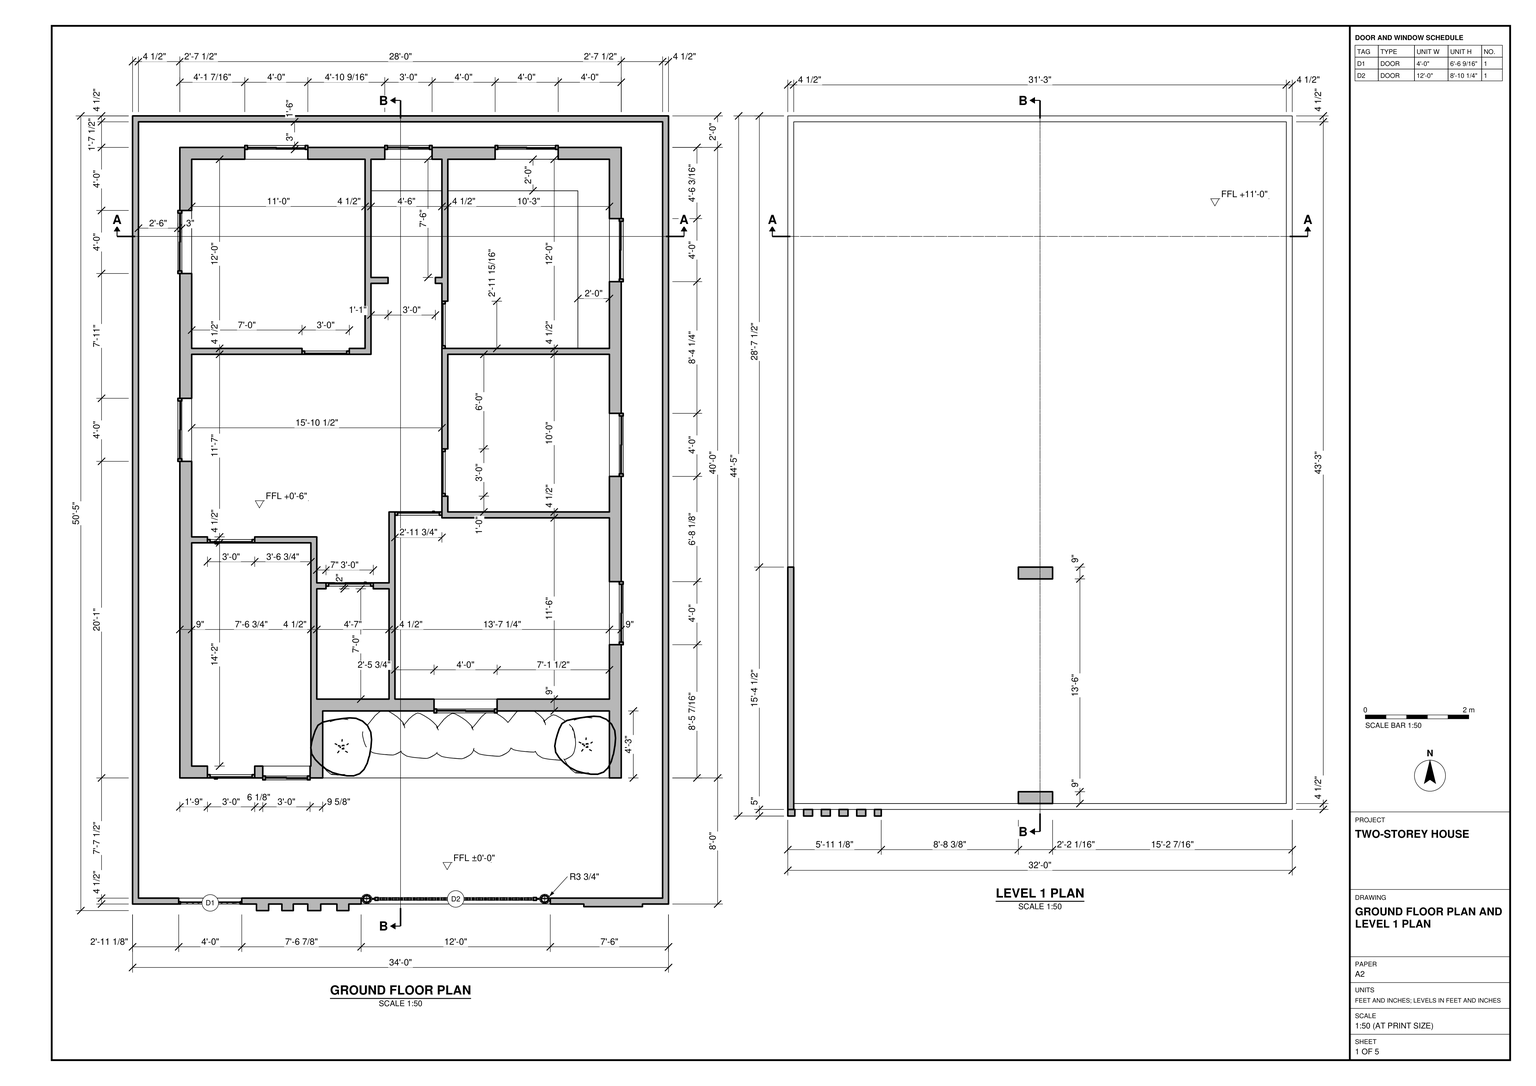
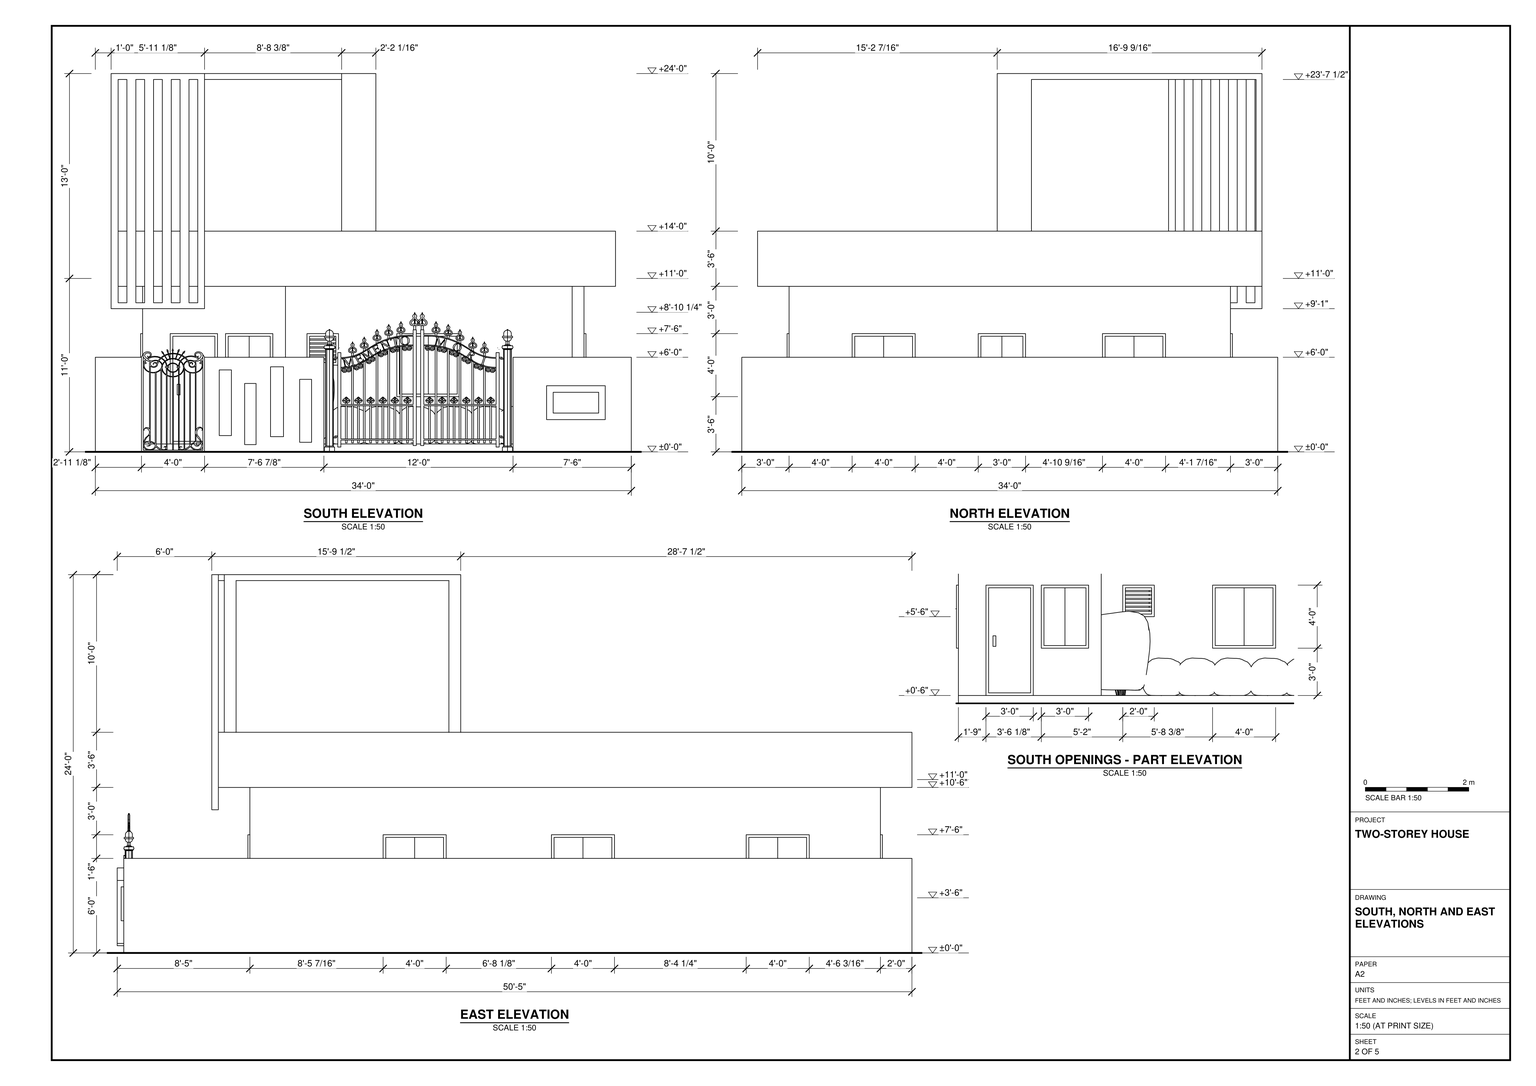
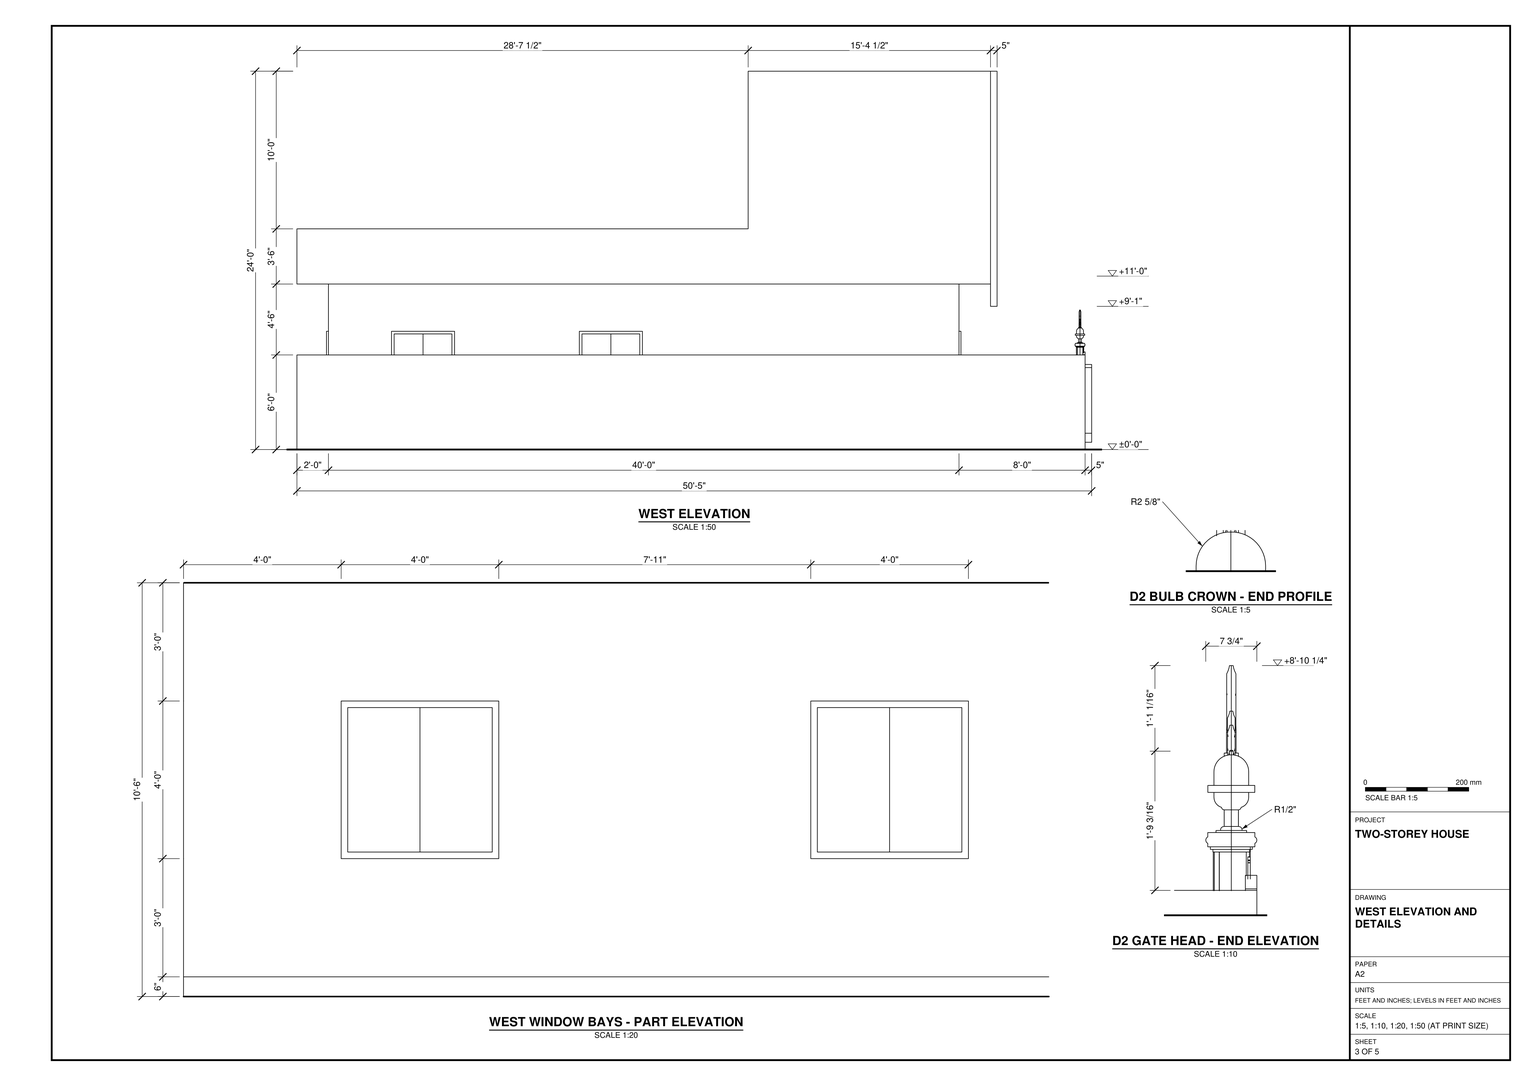
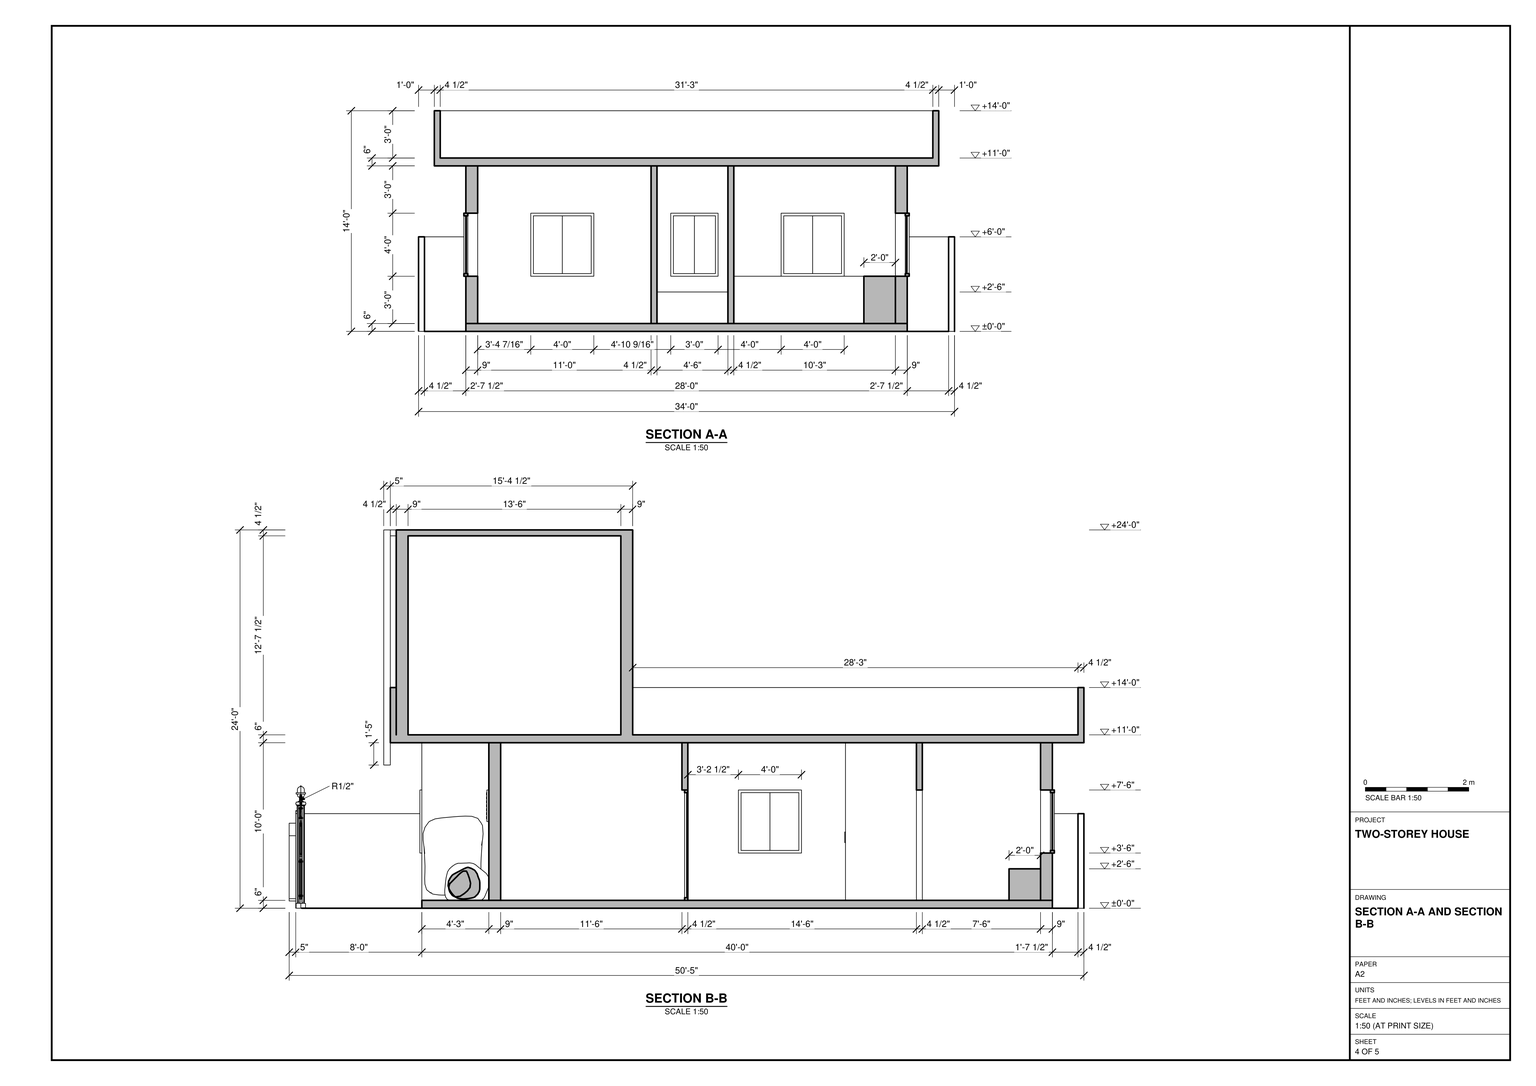
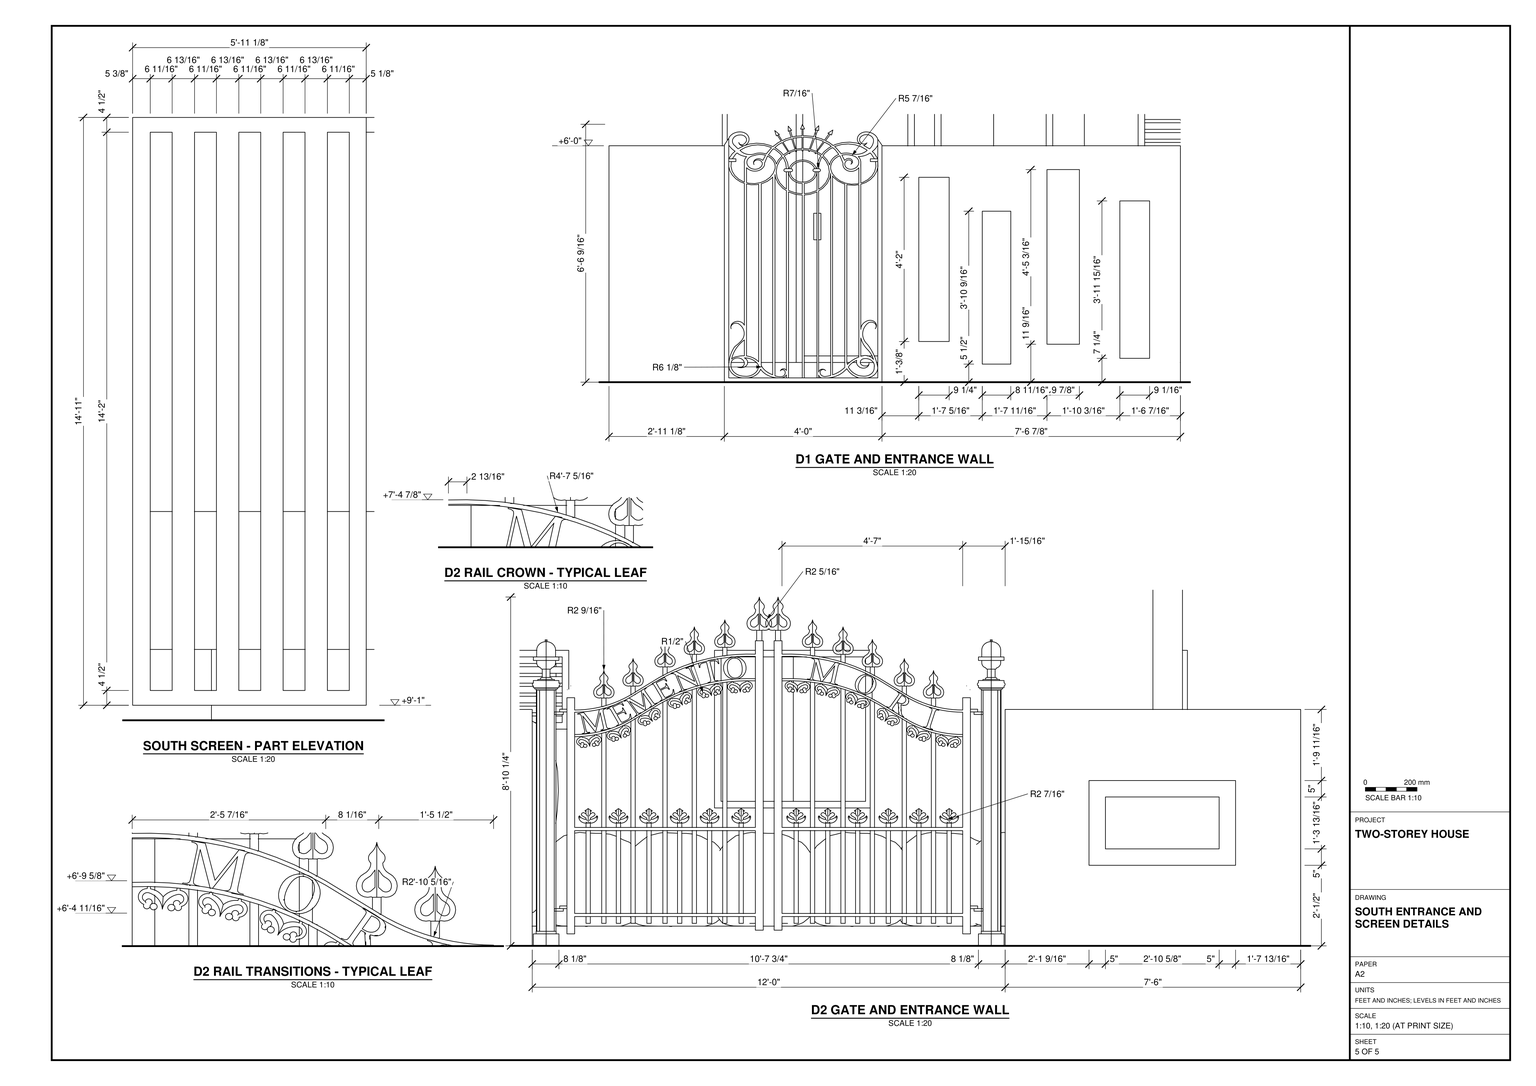
Build the house and its walled site in SketchUp using task_files/diagram_01.pdf. Work in feet and inches. The overall model is 34'-0" wide, 50'-5" deep and 24'-0" high. Use ±0'-0" as the ground datum and +11'-0" as the upper level. Set the house floor at +0'-6", above the forecourt.

Lay out the house behind the south boundary wall, leaving the forecourt, side clearances and rear setback shown in plan. Model the 9" exterior house walls and 4 1/2" interior partitions. Follow the room divisions, connecting doorways and framed window openings on the plan and elevations. At the front, distinguish the projecting entrance room from the recessed wall and planting strip beside it. Build the flat slab over the ground floor, the parapet around the open terrace and the tall frame with vertical fins at the southwest corner.

Model the narrow pedestrian gate and wider double gate in the south boundary wall. Use the elevations to shape the gate heads and place the panels in the adjoining wall. Decor and loose items, including the planting, may use any suitable library components. Keep shell elements such as walls, slabs and roof separate as groups or components, do the same for each furniture or joinery piece, and use components for repeated parts. Save one SketchUp model as output_files/two_storey_house_with_roof_terrace_and_gated_forecourt.skp.

# SketchUp Ruby script. Lengths in inches.
U = 1.inch
M = Sketchup.active_model
def pt(a) = Geom::Point3d.new(a.map { |v| v * U })
def face(e, loops, mat)
  f = e.add_face(loops[0].map { |a| pt(a) })
  loops[1..].each { |l| e.add_face(l.map { |a| pt(a) }).erase! }
  f.material = f.back_material = mat if mat
  f
end
# faces: each face lists its corners as indices into pts; further lists are holes
def faces(e, pts, list, mat = nil) = list.each { |f| face(e, (f[0].is_a?(Array) ? f : [f]).map { |l| l.map { |i| pts[i] } }, mat) }
# xy, xz, yz: faces in a plane at the given z, y or x. An outline is a flat list of corners, or four numbers for a rectangle; further outlines are holes
def ring(l) = l.size == 4 ? [[l[0], l[1]], [l[2], l[1]], [l[2], l[3]], [l[0], l[3]]] : l.each_slice(2).to_a
def flat(e, list, mat, &to3) = list.each { |f| face(e, (f[0].is_a?(Array) ? f : [f]).map { |l| ring(l).map { |u, v| to3.(u, v) } }, mat) }
def xy(e, z, list, mat = nil) = flat(e, list, mat) { |x, y| [x, y, z] }
def xz(e, y, list, mat = nil) = flat(e, list, mat) { |x, z| [x, y, z] }
def yz(e, x, list, mat = nil) = flat(e, list, mat) { |y, z| [x, y, z] }
def lines(e, pts, list) = list.each { |a, b| e.add_line(pt(pts[a]), pt(pts[b])) }
# prism: a flat outline (further loops are holes) pulled along v
def prism(e, loops, v, mat = nil)
  f = face(e, loops, mat); d = Geom::Vector3d.new(v.map { |x| x * U })
  f.pushpull(f.normal.samedirection?(d) ? d.length : -d.length)
end
def box(e, o, s, mat = nil) = prism(e, [[o, [o[0] + s[0], o[1], o[2]], [o[0] + s[0], o[1] + s[1], o[2]], [o[0], o[1] + s[1], o[2]]]], [0, 0, s[2]], mat)
def at(x, y, z, deg = 0) = Geom::Transformation.translation(pt([x, y, z])) * Geom::Transformation.rotation(ORIGIN, Z_AXIS, deg.degrees)
def axes(o, x, y, z) = Geom::Transformation.new([*x, 0, *y, 0, *z, 0, *pt(o).to_a, 1])
def part(name) = M.definitions.add(name)
# library, detail: a bought-in or finely detailed component or shape, given as its bounding box
def library(name, o, s) = part(name).tap { |d| box(d.entities, o, s) }
def detail(e, o, s) = box(e.add_group.entities, o, s)
def put(e, d, t, mat = nil) = e.add_instance(d, t).tap { |i| i.material = mat if mat }
def group(e, t, mat = nil) = e.add_group.tap { |g| g.transformation = t; g.material = mat if mat }.entities
root = M.entities
M.materials.add("Aluminium Black Anodized Fingerprints 15cm").color = [38, 38, 38]
M.materials.add("Glass Coated Blue").color = [0, 0, 0]
M.materials["Glass Coated Blue"].alpha = 0.35
M.materials.add("Grass C 200cm").color = [118, 136, 72]
M.materials.add("Tiles K01 100cm").color = [149, 135, 123]
M.materials.add("Wall Paint Fine Grain 01 Yellow 100cm").color = [207, 190, 139]
M.materials.add("Wall Paint Poised Taupe Satin 300cm").color = [140, 135, 132]
M.materials.add("Wood Dark 02 100cm").color = [99, 39, 19]
M.materials.add("Wood Dark Fine 18-26 80cm").color = [104, 73, 63]
c1 = library("Schefflera arboricola 001",[-25.43,-22.82,-0.1],[47.76,45.73,64.24])
c2 = library("Skimmia japonica Rubella 004",[-17.08,-16.64,-0.26],[33.2,34.59,28.81])
c3 = library("gate 533k",[0,0,0],[7.78,132.3,106.23])
c4 = library("gate 458k",[0,0,0],[53.16,1.75,104.71])
c5 = library("Dome Light",[-12,-12,0],[24,24,12])
c6 = part("Group\#6")
box(c6.entities,[0,0,0],[16,0.31,44])
c7 = part("Group\#8")
box(c7.entities,[0,-0.31,0],[20,0.31,2])
c8 = part("Group\#10")
box(c8.entities,[0,0,0],[22,0.31,44])
c9 = part("Group\#12")
box(c9.entities,[-0.31,0,0],[0.31,22,44])
c10 = part("Group\#14")
box(c10.entities,[-0.31,0,0],[0.31,22,44])
c11 = part("Group\#16")
box(c11.entities,[-0.31,0,0],[0.31,22,44])
c12 = part("Group\#18")
box(c12.entities,[0,-0.31,0],[22,0.31,44])
c13 = part("Group\#20")
box(c13.entities,[0,-0.31,0],[16,0.31,44])
c14 = part("Group\#22")
box(c14.entities,[0,-0.31,0],[22,0.31,44])
c15 = part("Group\#24")
box(c15.entities,[0,0,0],[0.31,22,44])
c16 = part("Group\#26")
box(c16.entities,[0,0,0],[0.31,22,44])
put(root,c1,at(159.61,124.73,0))
put(root,c1,at(345.35,125.97,0))
put(root,c2,at(192.09,135.07,0))
put(root,c2,at(217.83,132.5,0))
put(root,c2,at(244.47,132.23,0))
put(root,c2,at(273.02,134.13,0))
put(root,c2,at(299.28,137.3,0))
put(root,c2,at(321.125,131.1,0))
put(root,c3,axes([318,12.78,-6],[0,-1,0],[-1.08843,0,0],[0,0,1]))
put(root,c4,axes([35.125,5,-6],[0.90286,0,0],[0,1,0],[0,0,0.75]))
put(root,c5,axes([-74.51,70.32,-1.87],[2.55,0,0],[0,1,0],[0,0,2.51]))
g1 = group(root,at(36,101,0))
xy(g1,0,[[0,0,0,480,336,480,336,0,327,0,327,51,108.75,51,108.75,0,57,0,57,9,99.75,9,99.75,179,57,179,57,183.5,104.25,183.5,104.25,148.5,111.25,148.5,111.25,144,104.25,144,104.25,60,159.25,60,159.25,144,147.25,144,147.25,148.5,159.25,148.5,159.25,202.5,163.75,202.5,163.75,60,327,60,327,198,199.5,198,199.5,214.5,204,214.5,204,202.5,327,202.5,327,322.5,204,322.5,204,250.5,199.5,250.5,199.5,327,327,327,327,471,204,471,204,362.9375,199.5,362.9375,199.5,376.5,194.5,376.5,194.5,381,199.5,381,199.5,471,145.5,471,145.5,381,158.5,381,158.5,376.5,145.5,376.5,145.5,322.5,129,322.5,129,327,141,327,141,471,9,471,9,327,93,327,93,322.5,9,322.5,9,183.5,21,183.5,21,179,9,179,9,9,21,9,21,0]])
xy(g1,36,[[63.125,0,99.125,9],[193.5,51,241.5,60],[327,101.4375,336,149.4375],[327,229.5625,336,277.5625],[0,241,9,289],
  [327,377.8125,336,425.8125],[0,384,9,432],[49.4375,471,97.4375,480],[156,471,192,480],[240,471,288,480]])
xy(g1,60,[[125.125,51,149.125,60]])
xy(g1,84,[[21,0,57,9],[63.125,0,99.125,9],[125.125,51,149.125,60],[193.5,51,241.5,60],[327,101.4375,336,149.4375],
  [111.25,144,147.25,148.5],[21,179,57,183.5],[163.75,198,199.5,202.5],[199.5,214.5,204,250.5],[327,229.5625,336,277.5625],
  [0,241,9,289],[93,322.5,129,327],[199.5,327,204,362.9375],[158.5,376.5,194.5,381],[327,377.8125,336,425.8125],
  [0,384,9,432],[49.4375,471,97.4375,480],[156,471,192,480],[240,471,288,480]])
xy(g1,120,[[[0,0,108.75,0,108.75,51,327,51,327,0,336,0,336,480,0,480],[104.25,148.5,104.25,183.5,9,183.5,9,322.5,145.5,322.5,145.5,376.5,199.5,376.5,199.5,202.5,159.25,202.5,159.25,148.5],[163.75,60,327,198],[9,327,141,471],[204,327,327,471],[9,9,99.75,179],[204,202.5,327,322.5],[145.5,381,199.5,471],[104.25,60,159.25,144]]])
xz(g1,0,[[[0,0,21,0,21,84,57,84,57,0,108.75,0,108.75,120,0,120],[63.125,36,99.125,84]],[327,0,336,120]],"Wall Paint Fine Grain 01 Yellow 100cm")
xz(g1,9,[[[9,0,9,120,99.75,120,99.75,0,57,0,57,84,21,84,21,0],[63.125,36,99.125,84]]])
xz(g1,51,[[[108.75,0,327,120],[193.5,36,241.5,84],[125.125,60,149.125,84]]],"Wall Paint Fine Grain 01 Yellow 100cm")
xz(g1,60,[[[104.25,0,159.25,120],[125.125,60,149.125,84]],[[163.75,0,327,120],[193.5,36,241.5,84]]])
xz(g1,101.4375,[[327,36,336,84]])
xz(g1,144,[[104.25,0,111.25,0,111.25,84,147.25,84,147.25,0,159.25,0,159.25,120,104.25,120]])
xz(g1,148.5,[[104.25,0,104.25,120,159.25,120,159.25,0,147.25,0,147.25,84,111.25,84,111.25,0]])
xz(g1,149.4375,[[327,36,336,84]])
xz(g1,179,[[9,0,21,0,21,84,57,84,57,0,99.75,0,99.75,120,9,120]])
xz(g1,183.5,[[9,0,9,120,104.25,120,104.25,0,57,0,57,84,21,84,21,0]])
xz(g1,198,[[199.5,0,327,0,327,120,163.75,120,163.75,84,199.5,84]])
xz(g1,202.5,[[159.25,0,159.25,120,199.5,120,199.5,84,163.75,84,163.75,0],[204,0,327,120]])
xz(g1,214.5,[[199.5,0,204,84]])
xz(g1,229.5625,[[327,36,336,84]])
xz(g1,241,[[0,36,9,84]])
xz(g1,250.5,[[199.5,0,204,84]])
xz(g1,277.5625,[[327,36,336,84]])
xz(g1,289,[[0,36,9,84]])
xz(g1,322.5,[[9,0,93,0,93,84,129,84,129,0,145.5,0,145.5,120,9,120],[204,0,327,120]])
xz(g1,327,[[9,0,9,120,141,120,141,0,129,0,129,84,93,84,93,0],[199.5,0,199.5,84,204,84,204,120,327,120,327,0]])
xz(g1,362.9375,[[199.5,0,204,84]])
xz(g1,376.5,[[145.5,0,158.5,0,158.5,84,194.5,84,194.5,0,199.5,0,199.5,120,145.5,120]])
xz(g1,377.8125,[[327,36,336,84]])
xz(g1,381,[[145.5,0,145.5,120,199.5,120,199.5,0,194.5,0,194.5,84,158.5,84,158.5,0]])
xz(g1,384,[[0,36,9,84]])
xz(g1,425.8125,[[327,36,336,84]])
xz(g1,432,[[0,36,9,84]])
xz(g1,471,[[[9,0,141,120],[49.4375,36,97.4375,84]],[[145.5,0,199.5,120],[156,36,192,84]],[[204,0,327,120],[240,36,288,84]]])
xz(g1,480,[[[0,0,336,120],[240,36,288,84],[49.4375,36,97.4375,84],[156,36,192,84]]],"Wall Paint Fine Grain 01 Yellow 100cm")
yz(g1,0,[[[0,0,480,120],[384,36,432,84],[241,36,289,84]]],"Wall Paint Fine Grain 01 Yellow 100cm")
yz(g1,9,[[9,0,179,120],[[183.5,0,322.5,120],[241,36,289,84]],[[327,0,471,120],[384,36,432,84]]])
yz(g1,21,[[0,0,9,84],[179,0,183.5,84]])
yz(g1,49.4375,[[471,36,480,84]])
yz(g1,57,[[0,0,9,84],[179,0,183.5,84]])
yz(g1,63.125,[[0,36,9,84]])
yz(g1,93,[[322.5,0,327,84]])
yz(g1,97.4375,[[471,36,480,84]])
yz(g1,99.125,[[0,36,9,84]])
yz(g1,99.75,[[9,0,179,120]])
yz(g1,104.25,[[60,0,144,120],[148.5,0,183.5,120]])
yz(g1,108.75,[[0,0,51,120]],"Wall Paint Fine Grain 01 Yellow 100cm")
yz(g1,111.25,[[144,0,148.5,84]])
yz(g1,125.125,[[51,60,60,84]])
yz(g1,129,[[322.5,0,327,84]])
yz(g1,141,[[327,0,471,120]])
yz(g1,145.5,[[322.5,0,376.5,120],[381,0,471,120]])
yz(g1,147.25,[[144,0,148.5,84]])
yz(g1,149.125,[[51,60,60,84]])
yz(g1,156,[[471,36,480,84]])
yz(g1,158.5,[[376.5,0,381,84]])
yz(g1,159.25,[[60,0,144,120],[148.5,0,202.5,120]])
yz(g1,163.75,[[60,0,202.5,0,202.5,84,198,84,198,120,60,120]])
yz(g1,192,[[471,36,480,84]])
yz(g1,193.5,[[51,36,60,84]])
yz(g1,194.5,[[376.5,0,381,84]])
yz(g1,199.5,[[198,0,198,84,202.5,84,202.5,120,376.5,120,376.5,0,362.9375,0,362.9375,84,327,84,327,0,250.5,0,250.5,84,214.5,84,214.5,0],[381,0,471,120]])
yz(g1,204,[[202.5,0,214.5,0,214.5,84,250.5,84,250.5,0,322.5,0,322.5,120,202.5,120],[362.9375,0,471,0,471,120,327,120,327,84,362.9375,84]])
yz(g1,240,[[471,36,480,84]])
yz(g1,241.5,[[51,36,60,84]])
yz(g1,288,[[471,36,480,84]])
yz(g1,327,[[[60,0,198,120],[101.4375,36,149.4375,84]],[[202.5,0,322.5,120],[229.5625,36,277.5625,84]],[[327,0,471,120],[377.8125,36,425.8125,84]]])
yz(g1,327,[[0,0,51,120]],"Wall Paint Fine Grain 01 Yellow 100cm")
yz(g1,336,[[[0,0,480,120],[377.8125,36,425.8125,84],[101.4375,36,149.4375,84],[229.5625,36,277.5625,84]]],"Wall Paint Fine Grain 01 Yellow 100cm")
g2 = group(g1,at(21,0,0),"Aluminium Black Anodized Fingerprints 15cm")
prism(g2,[[[36,0,0],[36,0,84],[0,0,84],[0,0,0]],[[34,0,82],[34,0,2],[2,0,2],[2,0,82]]],[0,2.5,0],"Aluminium Black Anodized Fingerprints 15cm")
g3 = group(g1,at(23,0,2))
box(g3,[0,0,0],[32,0.71,80],"Wood Dark 02 100cm")
g4 = group(g3,at(3.34,0,35.37),"Aluminium Black Anodized Fingerprints 15cm")
box(g4,[0,-0.75,0],[2.1875,0.75,8.0625],"Aluminium Black Anodized Fingerprints 15cm")
g5 = group(g1,at(63.125,0,36))
prism(g5,[[[36,-1.5,0],[36,-1.5,48],[0,-1.5,48],[0,-1.5,0]],[[2,-1.5,46],[34,-1.5,46],[34,-1.5,2],[2,-1.5,2]]],[0,3,0],"Aluminium Black Anodized Fingerprints 15cm")
put(g5,c6,at(2,0,2),"Glass Coated Blue")
put(g5,c6,at(18,-0.31,2),"Glass Coated Blue")
g6 = group(g1,at(125.125,51,60))
prism(g6,[[[0,-1.5,0],[24,-1.5,0],[24,-1.5,24],[0,-1.5,24]],[[2,-1.5,2],[2,-1.5,22],[22,-1.5,22],[22,-1.5,2]]],[0,3,0],"Aluminium Black Anodized Fingerprints 15cm")
put(g6,c7,at(2,-1.5,20),"Glass Coated Blue")
put(g6,c7,at(2,-1.5,17),"Glass Coated Blue")
put(g6,c7,at(2,-1.5,14),"Glass Coated Blue")
put(g6,c7,at(2,-1.5,11),"Glass Coated Blue")
put(g6,c7,at(2,-1.5,8),"Glass Coated Blue")
put(g6,c7,at(2,-1.5,5),"Glass Coated Blue")
put(g6,c7,at(2,-1.5,2),"Glass Coated Blue")
g7 = group(g1,at(193.5,51,36))
prism(g7,[[[0,-1.5,0],[48,-1.5,0],[48,-1.5,48],[0,-1.5,48]],[[46,-1.5,2],[2,-1.5,2],[2,-1.5,46],[46,-1.5,46]]],[0,3,0],"Aluminium Black Anodized Fingerprints 15cm")
put(g7,c8,at(2,0.0625,2),"Glass Coated Blue")
put(g7,c8,at(24,-0.25,2),"Glass Coated Blue")
g8 = group(g1,at(336,101.4375,36))
prism(g8,[[[1.5,0,0],[1.5,48,0],[1.5,48,48],[1.5,0,48]],[[1.5,46,46],[1.5,46,2],[1.5,2,2],[1.5,2,46]]],[-3,0,0],"Aluminium Black Anodized Fingerprints 15cm")
put(g8,c9,at(0.125,2,2),"Glass Coated Blue")
put(g8,c9,at(0.44,24,2),"Glass Coated Blue")
g9 = group(g1,at(336,229.5625,36))
prism(g9,[[[1.5,0,0],[1.5,48,0],[1.5,48,48],[1.5,0,48]],[[1.5,46,2],[1.5,2,2],[1.5,2,46],[1.5,46,46]]],[-3,0,0],"Aluminium Black Anodized Fingerprints 15cm")
put(g9,c10,at(0,2,2),"Glass Coated Blue")
put(g9,c10,at(0.31,24,2),"Glass Coated Blue")
g10 = group(g1,at(336,377.8125,36))
prism(g10,[[[1.5,48,0],[1.5,48,48],[1.5,0,48],[1.5,0,0]],[[1.5,46,2],[1.5,2,2],[1.5,2,46],[1.5,46,46]]],[-3,0,0],"Aluminium Black Anodized Fingerprints 15cm")
put(g10,c11,at(-0.5625,2,2),"Glass Coated Blue")
put(g10,c11,at(-0.25,24,2),"Glass Coated Blue")
g11 = group(g1,at(240,480,36))
prism(g11,[[[48,1.5,0],[0,1.5,0],[0,1.5,48],[48,1.5,48]],[[46,1.5,46],[2,1.5,46],[2,1.5,2],[46,1.5,2]]],[0,-3,0],"Aluminium Black Anodized Fingerprints 15cm")
put(g11,c12,at(24,-0.3125,2),"Glass Coated Blue")
put(g11,c12,at(2,0,2),"Glass Coated Blue")
g12 = group(g1,at(156,480,36))
prism(g12,[[[0,1.5,0],[0,1.5,48],[36,1.5,48],[36,1.5,0]],[[34,1.5,46],[2,1.5,46],[2,1.5,2],[34,1.5,2]]],[0,-3,0],"Aluminium Black Anodized Fingerprints 15cm")
put(g12,c13,at(18,-0.1875,2),"Glass Coated Blue")
put(g12,c13,at(2,0.13,2),"Glass Coated Blue")
g13 = group(g1,at(49.4375,480,36))
prism(g13,[[[48,1.5,0],[0,1.5,0],[0,1.5,48],[48,1.5,48]],[[2,1.5,2],[46,1.5,2],[46,1.5,46],[2,1.5,46]]],[0,-3,0],"Aluminium Black Anodized Fingerprints 15cm")
put(g13,c14,at(24,-0.4375,2),"Glass Coated Blue")
put(g13,c14,at(2,-0.12,2),"Glass Coated Blue")
g14 = group(g1,at(0,384,36))
prism(g14,[[[-1.5,48,0],[-1.5,0,0],[-1.5,0,48],[-1.5,48,48]],[[-1.5,2,2],[-1.5,46,2],[-1.5,46,46],[-1.5,2,46]]],[3,0,0],"Aluminium Black Anodized Fingerprints 15cm")
put(g14,c15,at(0,24,2),"Glass Coated Blue")
put(g14,c15,at(-0.31,2,2),"Glass Coated Blue")
g15 = group(g1,at(0,241,36))
prism(g15,[[[-1.5,48,0],[-1.5,0,0],[-1.5,0,48],[-1.5,48,48]],[[-1.5,2,2],[-1.5,46,2],[-1.5,46,46],[-1.5,2,46]]],[3,0,0],"Aluminium Black Anodized Fingerprints 15cm")
put(g15,c16,at(0.1875,24,2),"Glass Coated Blue")
put(g15,c16,at(-0.13,2,2),"Glass Coated Blue")
g16 = group(g1,at(21,179,0))
prism(g16,[[[36,0,0],[36,0,84],[0,0,84],[0,0,0]],[[2,0,2],[2,0,82],[34,0,82],[34,0,2]]],[0,2.5,0])
g17 = group(g16,at(2,0,2))
box(g17,[0,0,0],[32,0.71,80])
g18 = group(g16,at(5.88,0,40.02))
box(g18,[0,-0.75,0],[1.8125,0.75,8.8125])
g19 = group(g1,at(93,322.5,0))
prism(g19,[[[36,2.5,0],[0,2.5,0],[0,2.5,84],[36,2.5,84]],[[34,2.5,82],[2,2.5,82],[2,2.5,2],[34,2.5,2]]],[0,-2.5,0])
g20 = group(g19,at(2,0,2))
box(g20,[0,0,0],[32,0.71,80])
g21 = group(g20,at(2.77,0,41.96))
box(g21,[0,-0.5625,0],[1.625,0.5625,8.0625])
g22 = group(g1,at(199.5,327,0))
prism(g22,[[[0,0,0],[0,0,84],[0,35.9375,84],[0,35.9375,0]],[[0,2,82],[0,2,2],[0,33.9375,2],[0,33.9375,82]]],[2.5,0,0])
g23 = group(g22,at(0,2,2))
box(g23,[0,0,0],[0.71,31.9375,80])
g24 = group(g23,at(0,27.84,43.88))
box(g24,[-0.3125,-1.4375,0],[0.3125,1.4375,7.0625])
g25 = group(g1,at(199.5,214.5,0))
prism(g25,[[[0,0,0],[0,0,84],[0,36,84],[0,36,0]],[[0,2,2],[0,34,2],[0,34,82],[0,2,82]]],[2.5,0,0])
g26 = group(g25,at(0,2,2))
box(g26,[0,0,0],[0.71,32,80])
g27 = group(g26,at(0,28.62,40.63))
box(g27,[-0.5625,-1.4375,0],[0.5625,1.4375,6.3125])
g28 = group(g1,at(163.75,202.5,0))
prism(g28,[[[0,0,0],[0,0,84],[35.75,0,84],[35.75,0,0]],[[33.75,0,82],[2,0,82],[2,0,2],[33.75,0,2]]],[0,-2.5,0])
g29 = group(g28,at(2,0,2))
box(g29,[0,-0.71,0],[31.75,0.71,80])
g30 = group(g28,at(28.73,0,36.67))
box(g30,[0,0,0],[1.25,0.4375,7.5])
g31 = group(g28,at(-52.5,-54,0))
prism(g31,[[[0,0,84],[36,0,84],[36,0,0],[0,0,0]],[[34,0,82],[2,0,82],[2,0,2],[34,0,2]]],[0,-2.5,0])
g32 = group(g31,at(2,0,2))
box(g32,[0,-0.71,0],[32,0.71,80])
g33 = group(g32,at(28.54,0,37.8))
box(g33,[-1.3125,0,0],[1.3125,0.4375,6.625])
g34 = group(g1,at(204,447,0))
prism(g34,[[[0,0,0],[0,24,0],[123,24,0],[123,-120,0],[99,-120,0],[99,0,0]]],[0,0,36])
g35 = group(g1,at(145.5,447,0))
box(g35,[0,0,0],[54,24,24])
g36 = group(root,at(62.39,280.71,37.76))
box(g36,[0,0,0],[1.125,0.375,5.375])
g37 = group(root,at(36,101,120))
xy(g37,0,[[-24,-24,360,504]],"Wall Paint Poised Taupe Satin 300cm")
xy(g37,6,[[[-19.5,-19.5,151.5,-19.5,151.5,-10.5,177.5625,-10.5,177.5625,-19.5,355.5,-19.5,355.5,499.5,-19.5,499.5],[151.5,151.5,177.5625,160.5]]])
xy(g37,42,[[-19.5,-24,360,-24,360,504,-24,504,-24,160.5,-19.5,160.5,-19.5,499.5,355.5,499.5,355.5,-19.5,-19.5,-19.5]],"Wall Paint Poised Taupe Satin 300cm")
xy(g37,157.5,[[-19.5,-24,-19.5,160.5,151.5,160.5,151.5,151.5,177.5625,151.5,177.5625,-10.5,151.5,-10.5,151.5,-24]],"Wall Paint Poised Taupe Satin 300cm")
xy(g37,162,[[-24,-24,151.5,-24,151.5,-19.5,177.5625,-19.5,177.5625,160.5,-24,160.5]],"Wall Paint Poised Taupe Satin 300cm")
xz(g37,-24,[[-24,0,360,42],[-24,42,-19.5,42,-19.5,157.5,151.5,157.5,151.5,162,-24,162]],"Wall Paint Poised Taupe Satin 300cm")
xz(g37,-19.5,[[-19.5,6,151.5,42],[151.5,6,177.5625,42],[177.5625,6,355.5,42],[151.5,42,177.5625,162]],"Wall Paint Poised Taupe Satin 300cm")
xz(g37,-10.5,[[151.5,6,177.5625,157.5]],"Wall Paint Poised Taupe Satin 300cm")
xz(g37,151.5,[[151.5,6,177.5625,157.5]],"Wall Paint Poised Taupe Satin 300cm")
xz(g37,160.5,[[151.5,6,151.5,157.5,-19.5,157.5,-19.5,42,-24,42,-24,162,177.5625,162,177.5625,6]],"Wall Paint Poised Taupe Satin 300cm")
xz(g37,499.5,[[-19.5,6,355.5,42]],"Wall Paint Poised Taupe Satin 300cm")
xz(g37,504,[[-24,0,360,42]],"Wall Paint Poised Taupe Satin 300cm")
yz(g37,-24,[[-24,0,-24,162,160.5,162,160.5,42,504,42,504,0]],"Wall Paint Poised Taupe Satin 300cm")
yz(g37,-19.5,[[-19.5,6,499.5,6,499.5,42,160.5,42,160.5,157.5,-24,157.5,-24,42,-19.5,42]],"Wall Paint Poised Taupe Satin 300cm")
yz(g37,151.5,[[-19.5,6,-10.5,157.5],[151.5,6,160.5,157.5],[-24,157.5,-19.5,162]],"Wall Paint Poised Taupe Satin 300cm")
yz(g37,177.5625,[[-19.5,6,-10.5,6,-10.5,157.5,151.5,157.5,151.5,6,160.5,6,160.5,162,-19.5,162]],"Wall Paint Poised Taupe Satin 300cm")
yz(g37,355.5,[[-19.5,6,499.5,42]],"Wall Paint Poised Taupe Satin 300cm")
yz(g37,360,[[-24,0,504,42]],"Wall Paint Poised Taupe Satin 300cm")
g38 = group(root,at(36,101,-6))
xy(g38,0,[[0,0,336,480]])
xy(g38,6,[[0,0,336,480]],"Grass C 200cm")
xz(g38,0,[[0,0,336,6]])
xz(g38,480,[[0,0,336,6]])
yz(g38,0,[[0,0,480,6]])
yz(g38,336,[[0,0,480,6]])
g39 = group(root,at(0,5,-6))
xy(g39,0,[[83.125,0,174,4.5]])
xy(g39,0,[[4.5,4.5,403.5,595.5]],"Tiles K01 100cm")
xy(g39,5.5,[[113.67,-5,122.35,0]],"Wood Dark Fine 18-26 80cm")
xy(g39,7.26,[[155.56,-5,164.62,0]],"Wood Dark Fine 18-26 80cm")
xy(g39,11.56,[[133.37,-5,143.24,0]],"Wood Dark Fine 18-26 80cm")
xy(g39,12.38,[[94.34,-5,103.59,0]],"Wood Dark Fine 18-26 80cm")
xy(g39,24.53,[[343.54,-2,388.17,0]],"Wood Dark Fine 18-26 80cm")
xy(g39,29.53,[[348.54,-2,383.17,3]],"Wood Dark Fine 18-26 80cm")
xy(g39,45.34,[[348.54,-2,383.17,3]],"Wood Dark Fine 18-26 80cm")
xy(g39,50.34,[[343.54,-2,388.17,0]],"Wood Dark Fine 18-26 80cm")
xy(g39,52.07,[[113.67,-5,122.35,0]],"Wood Dark Fine 18-26 80cm")
xy(g39,55.2,[[155.56,-5,164.62,0]],"Wood Dark Fine 18-26 80cm")
xy(g39,62.38,[[94.34,-5,103.59,0]],"Wood Dark Fine 18-26 80cm")
xy(g39,64.75,[[133.37,-5,143.24,0]],"Wood Dark Fine 18-26 80cm")
xy(g39,72,[[0,0,35.125,0,35.125,4.5,4.5,4.5,4.5,595.5,403.5,595.5,403.5,4.5,318,4.5,318,0,408,0,408,600,0,600],[83.125,0,174,4.5]],"Wall Paint Poised Taupe Satin 300cm")
xz(g39,-5,[[113.67,5.5,122.35,52.07],[155.56,7.26,164.62,55.2],[133.37,11.56,143.24,64.75],[94.34,12.38,103.59,62.38]],"Wood Dark Fine 18-26 80cm")
xz(g39,-2,[[[343.54,24.53,388.17,50.34],[348.54,29.53,383.17,45.34]]],"Wood Dark Fine 18-26 80cm")
xz(g39,0,[[0,0,35.125,72],[[83.125,0,174,72],[133.37,11.56,143.24,64.75],[94.34,12.38,103.59,62.38],[155.56,7.26,164.62,55.2],[113.67,5.5,122.35,52.07]],[[318,0,408,72],[343.54,24.53,388.17,50.34]]],"Wall Paint Poised Taupe Satin 300cm")
xz(g39,3,[[348.54,29.53,383.17,45.34]],"Wood Dark Fine 18-26 80cm")
xz(g39,4.5,[[4.5,0,35.125,72]])
xz(g39,4.5,[[83.125,0,174,72],[318,0,403.5,72]],"Wall Paint Poised Taupe Satin 300cm")
xz(g39,595.5,[[4.5,0,403.5,72]],"Wall Paint Poised Taupe Satin 300cm")
xz(g39,600,[[0,0,408,72]],"Wall Paint Poised Taupe Satin 300cm")
yz(g39,0,[[0,0,600,72]],"Wall Paint Poised Taupe Satin 300cm")
yz(g39,4.5,[[4.5,0,595.5,72]],"Wall Paint Poised Taupe Satin 300cm")
yz(g39,35.125,[[0,0,4.5,72]],"Wall Paint Poised Taupe Satin 300cm")
yz(g39,83.125,[[0,0,4.5,72]],"Wall Paint Poised Taupe Satin 300cm")
yz(g39,94.34,[[-5,12.38,0,62.38]],"Wood Dark Fine 18-26 80cm")
yz(g39,103.59,[[-5,12.38,0,62.38]],"Wood Dark Fine 18-26 80cm")
yz(g39,113.67,[[-5,5.5,0,52.07]],"Wood Dark Fine 18-26 80cm")
yz(g39,122.35,[[-5,5.5,0,52.07]],"Wood Dark Fine 18-26 80cm")
yz(g39,133.37,[[-5,11.56,0,64.75]],"Wood Dark Fine 18-26 80cm")
yz(g39,143.24,[[-5,11.56,0,64.75]],"Wood Dark Fine 18-26 80cm")
yz(g39,155.56,[[-5,7.26,0,55.2]],"Wood Dark Fine 18-26 80cm")
yz(g39,164.62,[[-5,7.26,0,55.2]],"Wood Dark Fine 18-26 80cm")
yz(g39,174,[[0,0,4.5,72]],"Wall Paint Poised Taupe Satin 300cm")
yz(g39,318,[[0,0,4.5,72]])
yz(g39,343.54,[[-2,24.53,0,50.34]],"Wood Dark Fine 18-26 80cm")
yz(g39,348.54,[[-2,29.53,3,45.34]],"Wood Dark Fine 18-26 80cm")
yz(g39,383.17,[[-2,29.53,3,45.34]],"Wood Dark Fine 18-26 80cm")
yz(g39,388.17,[[-2,24.53,0,50.34]],"Wood Dark Fine 18-26 80cm")
yz(g39,403.5,[[4.5,0,595.5,72]],"Wall Paint Poised Taupe Satin 300cm")
yz(g39,408,[[0,0,600,72]],"Wall Paint Poised Taupe Satin 300cm")
p = [[35.125,0,0],[83.125,0,0],[174,0,0],[318,0,0]]
lines(g39,p,[[0,1],[2,3]])
g40 = group(root,at(12,77,120),"Wood Dark Fine 18-26 80cm")
prism(g40,[[[71.125,0,162],[71.125,0,-17],[0,0,-17],[0,0,162]],[[18.85,0,157.5],[18.85,0,-12.5],[25.52,0,-12.5],[25.52,0,157.5]],[[32.33,0,157.5],[32.33,0,-12.5],[39,0,-12.5],[39,0,157.5]],[[45.82,0,157.5],[45.82,0,-12.5],[52.49,0,-12.5],[52.49,0,157.5]],[[59.3,0,157.5],[59.3,0,-12.5],[65.97,0,-12.5],[65.97,0,157.5]],[[5.36,0,157.5],[5.36,0,-12.5],[12.03,0,-12.5],[12.03,0,157.5]]],[0,-5,0],"Wood Dark Fine 18-26 80cm")
